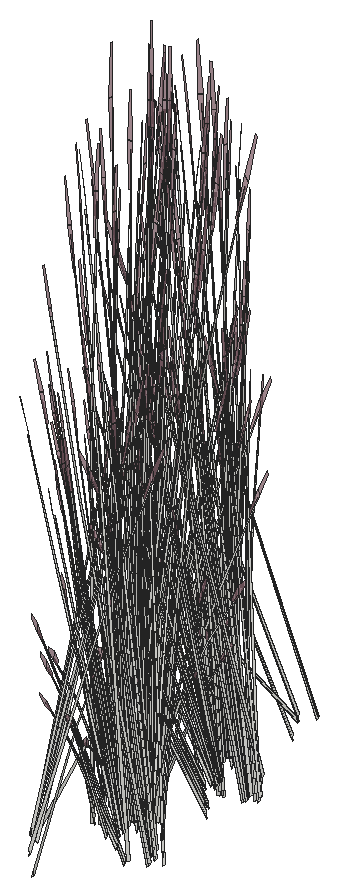
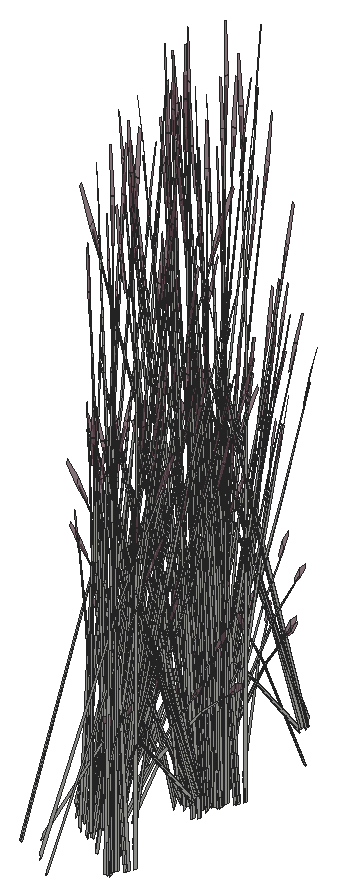
# SketchUp Ruby script. Lengths in inches.
U = 1.inch
M = Sketchup.active_model
def pt(a) = Geom::Point3d.new(a.map { |v| v * U })
def face(e, loops, mat)
  f = e.add_face(loops[0].map { |a| pt(a) })
  loops[1..].each { |l| e.add_face(l.map { |a| pt(a) }).erase! }
  f.material = f.back_material = mat if mat
  f
end
# faces: each face lists its corners as indices into pts; further lists are holes
def faces(e, pts, list, mat = nil) = list.each { |f| face(e, (f[0].is_a?(Array) ? f : [f]).map { |l| l.map { |i| pts[i] } }, mat) }
# xy, xz, yz: faces in a plane at the given z, y or x. An outline is a flat list of corners, or four numbers for a rectangle; further outlines are holes
def ring(l) = l.size == 4 ? [[l[0], l[1]], [l[2], l[1]], [l[2], l[3]], [l[0], l[3]]] : l.each_slice(2).to_a
def flat(e, list, mat, &to3) = list.each { |f| face(e, (f[0].is_a?(Array) ? f : [f]).map { |l| ring(l).map { |u, v| to3.(u, v) } }, mat) }
def xy(e, z, list, mat = nil) = flat(e, list, mat) { |x, y| [x, y, z] }
def xz(e, y, list, mat = nil) = flat(e, list, mat) { |x, z| [x, y, z] }
def yz(e, x, list, mat = nil) = flat(e, list, mat) { |y, z| [x, y, z] }
def lines(e, pts, list) = list.each { |a, b| e.add_line(pt(pts[a]), pt(pts[b])) }
# prism: a flat outline (further loops are holes) pulled along v
def prism(e, loops, v, mat = nil)
  f = face(e, loops, mat); d = Geom::Vector3d.new(v.map { |x| x * U })
  f.pushpull(f.normal.samedirection?(d) ? d.length : -d.length)
end
def box(e, o, s, mat = nil) = prism(e, [[o, [o[0] + s[0], o[1], o[2]], [o[0] + s[0], o[1] + s[1], o[2]], [o[0], o[1] + s[1], o[2]]]], [0, 0, s[2]], mat)
def at(x, y, z, deg = 0) = Geom::Transformation.translation(pt([x, y, z])) * Geom::Transformation.rotation(ORIGIN, Z_AXIS, deg.degrees)
def axes(o, x, y, z) = Geom::Transformation.new([*x, 0, *y, 0, *z, 0, *pt(o).to_a, 1])
def part(name) = M.definitions.add(name)
# library, detail: a bought-in or finely detailed component or shape, given as its bounding box
def library(name, o, s) = part(name).tap { |d| box(d.entities, o, s) }
def detail(e, o, s) = box(e.add_group.entities, o, s)
def put(e, d, t, mat = nil) = e.add_instance(d, t).tap { |i| i.material = mat if mat }
def group(e, t, mat = nil) = e.add_group.tap { |g| g.transformation = t; g.material = mat if mat }.entities
root = M.entities
M.materials.add("LightPink_Translucent").color = [144, 107, 117]
M.materials["LightPink_Translucent"].alpha = 0.75
c1 = part("blade")
p = [[2.15,0.21,22],[0,0.17,0],[0.09,0.45,0],[2.18,0.31,22],[2.29,0.31,22],[0.38,0.45,0],
  [2.48,0.24,33],[2.49,0.24,33],[2.48,0.22,33]]
faces(c1.entities,p,[[0,1,2,3],[4,5,2,3],[6,3,4,7],[8,0,3,6]])
c2 = part("seeds")
p = [[0.3,-0.1,1.38],[-0.01,-0.03,1.59],[-0.01,-0.03,0.03],[0.14,-0.07,-0.07],[0.29,-0.03,3],[0.15,0.01,3.11]]
faces(c2.entities,p,[[0,1,2,3],[1,0,4,5]],"LightPink_Translucent")
c3 = part("blade with seeds")
put(c3.entities,c1,at(0,0,0))
put(c3.entities,c2,axes([2.4,0.25,30.99],[1.5799,-0.05474,1.17369],[-0.12525,1.92788,0.29478],[-0.07173,-0.02425,1.56792]))
put(root,c3,axes([404.54,32.26,-9.59],[-0.14537,0.11002,1.33163],[-0.43536,-0.19256,-0.28638],[0.0807,-0.23948,0.56934]))
put(root,c3,axes([403.38,24.93,-7.3125],[0.50045,-0.25306,-0.11324],[0.24593,0.44915,-0.62851],[0.06603,0.18927,0.95501]))
put(root,c3,axes([408.26,29.88,-9.83],[-0.47569,0.45698,0.2864],[-0.47598,-0.45217,-0.33981],[-0.01661,-0.12977,1.53541]))
put(root,c3,axes([407.6,27.93,-7.62],[0.03791,0.05424,1.65179],[-0.18278,0.48761,-0.15608],[-0.18511,0.00353,0.29231]))
put(root,c3,axes([403.47,25.03,-10.61],[0.08277,-0.02958,1.6421],[0.49786,0.16279,-0.25086],[0.01456,0.18348,0.2797]))
put(root,c3,axes([408.12,28.9375,-7.64],[-0.37135,0.36005,-0.47583],[-0.32522,-0.38035,-0.36857],[-0.18868,-0.05478,0.91046]))
put(root,c3,axes([408.39,28.78,-7.3],[0.29098,0.34031,0.32977],[-0.33226,0.32215,-0.42575],[-0.16881,-0.04902,0.81462]))
put(root,c3,axes([407.28,29.41,-9.42],[0.3265,-0.03889,1.06958],[-0.20711,0.3427,0.78586],[-0.16135,-0.05141,0.23558]))
put(root,c3,axes([404.89,33.07,-7.36],[0.01331,-0.50278,-0.66157],[0.56035,0.03377,0.07984],[0.05914,-0.213,0.93586]))
put(root,c3,axes([403.8125,24.91,-7.64],[0.50273,0.13626,-0.47583],[-0.17232,0.46717,-0.36857],[0.0461,0.18809,0.91046]))
put(root,c3,axes([404.1,23.94,-8.39],[-0.1169,-0.17452,1.59586],[0.54019,-0.14692,0.12904],[0.12209,0.27397,0.68222]))
put(root,c3,axes([405.67,32.29,-7.61],[-0.00494,-0.10818,1.62908],[-0.41695,-0.31265,-0.25764],[0.06446,-0.18952,0.13065]))
put(root,c3,axes([405.5625,31.9,-7.62],[-0.05194,0.04152,1.65179],[-0.50886,-0.14007,-0.15608],[-0.01842,-0.18118,0.29231]))
put(root,c3,axes([408.31,28.56,-7.3125],[-0.02738,0.55277,-0.11324],[-0.51847,-0.01511,-0.62851],[-0.19968,-0.0384,0.95501]))
put(root,c3,axes([403.58,25.19,-7.78],[-0.15418,0.41799,-0.32977],[-0.44981,-0.12192,0.42575],[0.04124,0.16829,0.81462]))
put(root,c3,axes([404,31.38,-9.42],[0.06561,0.31695,1.06958],[-0.36394,-0.17555,0.78586],[0.03916,-0.16229,0.23558]))
put(root,c3,axes([404.78,32.91,-7.64],[-0.3661,-0.36521,-0.47583],[0.38674,-0.31985,-0.36857],[0.0557,-0.18556,0.91046]))
put(root,c3,axes([409.23,30.75,-10.08],[-0.53199,-0.08911,-0.58063],[0.11226,-0.54969,-0.15239],[-0.15876,-0.06661,1.28164]))
put(root,c3,axes([403.98,32.36,-7.59],[0.50393,0.1421,0.447],[-0.17232,0.46717,0.36857],[-0.03028,-0.18372,0.92496]))
put(root,c3,axes([403.63,24.82,-7.36],[0.24409,0.44196,-0.66157],[-0.50245,0.2463,0.07984],[0.05708,0.21354,0.93586]))
put(root,c3,axes([405.16,33.1,-7.3125],[-0.56206,-0.02693,-0.11324],[0.01536,-0.50991,-0.62851],[0.03904,-0.19638,0.95501]))
put(root,c3,axes([405.125,32.77,-7.78],[0.34603,-0.28618,-0.32977],[0.32756,0.32677,0.42575],[0.04984,-0.16603,0.81462]))
put(root,c3,axes([404.11,32.33,-7.6],[0.37684,-0.18473,0.05988],[0.18445,0.33686,0.47138],[-0.03639,-0.14849,0.71878]))
put(root,c3,axes([403.26,25.93,-7.61],[0.06483,0.08753,1.62908],[0.52315,0.03439,-0.25764],[0.05261,0.19303,0.13065]))
put(root,c3,axes([407.57,29.72,-7.59],[0.14449,-0.4956,0.447],[0.47502,0.16947,0.36857],[-0.1868,0.02978,0.92496]))
put(root,c3,axes([407.53,29.59,-7.6],[-0.18783,-0.37061,0.05988],[0.34252,-0.1814,0.47138],[-0.15099,0.03579,0.71878]))
put(root,c3,axes([407.52,29.97,-10.61],[0.01297,0.08566,1.6421],[-0.26146,0.44735,-0.25086],[-0.18572,-0.02255,0.2797]))
put(root,c3,axes([408.67,31.59,-10.11],[-0.12013,-0.47362,-0.28847],[0.47712,-0.13449,0.28847],[-0.09619,-0.05462,1.29413]))
put(root,c3,axes([408.53,31.79,-10.12],[-0.47863,-0.27177,-0.46235],[0.28609,-0.48733,0],[-0.10901,-0.0619,1.46668]))
put(root,c3,axes([409.83,30.83,-9.52],[-0.51635,0.36087,-0.27094],[-0.34336,-0.5099,-0.46562],[-0.1274,-0.05178,1.4872]))
put(root,c3,axes([405.125,32.88,-7.59],[0.36417,0.37086,0.447],[-0.38674,0.31985,0.36857],[0.06718,-0.174,0.92496]))
put(root,c3,axes([405.26,32.92,-7.6],[0.42027,0.02533,0.05988],[-0.01152,0.38243,0.47138],[0.04398,-0.14649,0.71878]))
put(root,c3,axes([404.94,33.18,-7.3],[-0.34603,0.28618,0.32977],[-0.32756,-0.32677,-0.42575],[0.04984,-0.16603,0.81462]))
put(root,c3,axes([402.67,32.7,-9.79],[-0.31974,-0.54466,0],[0.53494,-0.30375,-0.48057],[0.12184,-0.06918,1.52448]))
put(root,c3,axes([407.92,29.73,-7.3],[0.42502,0.15163,0.32977],[-0.12396,0.44238,-0.42575],[-0.17112,0.04056,0.81462]))
put(root,c3,axes([403.1,32.62,-10.12],[0.47863,-0.27177,-0.46235],[0.28609,0.48733,0],[0.10901,-0.0619,1.46668]))
put(root,c3,axes([403.67,33.73,-10.08],[0.34446,-0.40855,-0.58063],[0.42791,0.37046,-0.15239],[0.13803,-0.10191,1.28164]))
put(root,c3,axes([407.76,30,-7.64],[-0.13855,0.49442,-0.47583],[-0.47502,-0.16947,-0.36857],[-0.19125,0.04534,0.91046]))
put(root,c3,axes([407.74,29.58,-7.3125],[0.25732,0.49218,-0.11324],[-0.45669,0.24187,-0.62851],[-0.19245,0.06494,0.95501]))
put(root,c3,axes([408.82,32.12,-9.79],[-0.31974,0.54466,0],[-0.53494,-0.30375,-0.48057],[-0.12184,-0.06918,1.52448]))
put(root,c3,axes([403.29,34.2,-9.52],[-0.05959,-0.62022,-0.27094],[0.62068,-0.0375,-0.46562],[0.1093,-0.08261,1.4872]))
put(root,c3,axes([405.54,34.0625,-7.3],[-0.44516,0.07768,0.32977],[-0.11755,-0.44407,-0.42575],[0.12757,-0.11927,0.81462]))
put(root,c3,axes([403.21,32.83,-10.11],[0.47712,0.13449,-0.28847],[-0.12013,0.47362,0.28847],[0.09619,-0.05462,1.29413]))
put(root,c3,axes([407.68,30.96,-7.59],[-0.12683,-0.50025,0.447],[0.49754,-0.08682,0.36857],[-0.14663,0.11765,0.92496]))
put(root,c3,axes([407.58,30.86,-7.6],[-0.35109,-0.22859,0.05988],[0.2044,-0.32553,0.47138],[-0.11256,0.10524,0.71878]))
put(root,c3,axes([403.375,34.69,-9.73],[0.57623,0.26344,0.22409],[-0.27732,0.5474,0.46562],[0,-0.12618,1.49497]))
put(root,c3,axes([407.99,30.79,-7.3],[0.44516,-0.07768,0.32977],[0.11755,0.44407,-0.42575],[-0.12757,0.11927,0.81462]))
put(root,c3,axes([406.27,30.59,-7.62],[0.06527,0.01458,1.65179],[0.20191,0.48025,-0.15608],[-0.1336,0.12605,0.29231]))
put(root,c3,axes([406.82,32.12,-9.42],[0.21313,-0.24635,1.06958],[0.0841,0.38999,0.78586],[-0.15402,0.06983,0.23558]))
put(root,c3,axes([407.625,31.05,-7.78],[-0.44516,0.07768,-0.32977],[-0.11755,-0.44407,0.42575],[-0.12757,0.11927,0.81462]))
put(root,c3,axes([403.1875,34.32,-9.47],[-0.55535,0.03355,0.41661],[-0.05022,-0.55698,-0.2005],[0.09942,-0.05645,1.33761]))
put(root,c3,axes([406.98,32.05,-6.74],[0.45129,0.14509,-0.06041],[-0.13882,0.44656,-0.27392],[-0.07381,0.0678,0.90349]))
put(root,c3,axes([410.18,31.22,-10.08],[-0.34446,0.40855,-0.58063],[-0.42791,-0.37046,-0.15239],[-0.13803,0.10191,1.28164]))
put(root,c3,axes([403.97,34.57,-9.95],[0,-0.62892,0],[0.63949,0,0],[0,0,1.6711]))
put(root,c3,axes([404.75,33.12,-9.69],[-0.47863,-0.27177,0.46235],[0.28609,-0.48733,0],[0.10901,0.0619,1.46668]))
put(root,c3,axes([403.67,34.18,-9.8],[-0.42403,0.49328,0.42607],[-0.50377,-0.43543,0.16719],[0.10223,-0.04923,1.47927]))
put(root,c3,axes([407.76,30.75,-7.3125],[0.47307,0.29971,-0.11324],[-0.27254,0.43404,-0.62851],[-0.13365,0.15087,0.95501]))
put(root,c3,axes([402.93,33.37,-9.7],[-0.14774,0.54019,0.16428],[-0.54062,-0.15287,0.32672],[0.09339,-0.00263,1.49371]))
put(root,c3,axes([408.36,38.75,-8.39],[0.1169,0.17452,1.59586],[-0.54019,0.14692,0.12904],[-0.12209,-0.27397,0.68222]))
put(root,c3,axes([408.39,30.62,-8.39],[0.12773,-0.16701,1.59586],[0.32252,0.4508,0.12904],[-0.22121,0.20529,0.68222]))
put(root,c3,axes([404.06,33.97,-9.5625],[0.09866,-0.48509,0.13483],[0.48202,0.0842,-0.38503],[0.08772,0.04981,1.18024]))
put(root,c3,axes([407.99,31.11,-7.64],[0.13138,0.49631,-0.47583],[-0.49754,0.08682,-0.36857],[-0.14258,0.13331,0.91046]))
put(root,c3,axes([403.85,34.09,-9.47],[-0.30722,-0.45622,0.41661],[0.46535,-0.32126,-0.2005],[0.09942,0.05645,1.33761]))
put(root,c3,axes([408.21,38.28,-9.59],[-0.03097,0.17781,1.33163],[-0.45273,0.14885,-0.28638],[-0.10583,-0.22982,0.56934]))
put(root,c3,axes([408.27,31.94,-7.6],[-0.42027,-0.02533,0.05988],[0.01152,-0.38243,0.47138],[-0.04398,0.14649,0.71878]))
put(root,c3,axes([407.38,32.37,-10.61],[0.0686,0.0543,1.6421],[0.11632,0.50315,-0.25086],[-0.15204,0.10729,0.2797]))
put(root,c3,axes([408.41,31.97,-7.59],[-0.36417,-0.37086,0.447],[0.38674,-0.31985,0.36857],[-0.06718,0.174,0.92496]))
put(root,c3,axes([404.01,34.125,-9.52],[0.51635,-0.36087,-0.27094],[0.34336,0.5099,-0.46562],[0.1274,0.05178,1.4872]))
put(root,c3,axes([404.4,34.72,-9.95],[0.57217,0,0],[0,0.56272,0],[0,0,1.66132]))
put(root,c3,axes([404.57,33.4,-9.7],[-0.54955,0.14427,0.16428],[-0.1357,-0.53689,0.32672],[0.04901,0.07823,1.49371]))
put(root,c3,axes([405.18,33.37,-10.11],[0.12013,0.47362,-0.28847],[-0.47712,0.13449,0.28847],[0.09619,0.05462,1.29413]))
put(root,c3,axes([408.3,31.03,-8.39],[0.09522,-0.18683,1.59586],[0.39947,0.38663,0.12904],[-0.18021,0.24097,0.68222]))
put(root,c3,axes([404.22,34.43,-9.78],[-0.64638,-0.11452,0.45814],[0.13155,-0.64678,0.17978],[0.09446,0.06245,1.59061]))
put(root,c3,axes([408.72,37.34,-7.62],[-0.00954,0.06515,1.65179],[-0.47055,0.23645,-0.15608],[-0.13847,-0.12087,0.29231]))
put(root,c3,axes([408.41,32.08,-7.78],[-0.34603,0.28618,-0.32977],[-0.32756,-0.32677,0.42575],[-0.04984,0.16603,0.81462]))
put(root,c3,axes([407.21,32,-7.61],[-0.01271,0.10756,1.62908],[0.36076,0.37419,-0.25764],[-0.09444,0.17695,0.13065]))
put(root,c3,axes([404.33,35.96,-9.97],[0.53691,-0.18442,-0.17877],[0.18866,0.53125,0.00007],[0.05927,-0.02038,1.61933]))
put(root,c3,axes([408.62,38.49,-7.26],[0.56969,-0.13971,0.50064],[0.09887,0.54803,0.4128],[-0.13398,-0.16152,1.03595]))
put(root,c3,axes([404.39,34.96,-9.9375],[0.35699,0.35109,0],[-0.35699,0.35109,0],[0,0,1.57621]))
put(root,c3,axes([405.36,34.8,-9.7],[-0.40181,-0.39593,0.16428],[0.40492,-0.38402,0.32672],[-0.04438,0.08086,1.49371]))
put(root,c3,axes([408.06,38,-9.42],[0.26677,0.18918,1.06958],[-0.38851,0.11372,0.78586],[-0.08313,-0.14539,0.23558]))
put(root,c3,axes([408.7,39,-7.36],[-0.43608,-0.26272,-0.66157],[0.30991,-0.46038,0.07984],[-0.158,-0.15687,0.93586]))
put(root,c3,axes([408.55,38.65,-7.78],[-0.07899,-0.43781,-0.32977],[0.45153,-0.11561,0.42575],[-0.12128,-0.12546,0.81462]))
put(root,c3,axes([404.39,34.55,-9.47],[0.24813,-0.48978,0.41661],[0.51557,0.23571,-0.2005],[0,0.1129,1.33761]))
put(root,c3,axes([404.29,34.83,-9.87],[0,0.62861,-0.05249],[-0.63949,0,0],[0,0.01975,1.67027]))
put(root,c3,axes([404.34,34.38,-9.94],[0.30722,0.45622,-0.41661],[-0.46535,0.32126,0.2005],[0.09942,0.05645,1.33761]))
put(root,c3,axes([408.75,38.61,-7.6],[0.23243,-0.34529,0.05988],[0.331,0.20103,0.47138],[-0.10701,-0.1107,0.71878]))
put(root,c3,axes([407.85,38.57,-10.61],[-0.04954,0.0716,1.6421],[-0.50062,0.15438,-0.25086],[-0.12094,-0.14044,0.2797]))
put(root,c3,axes([405.6875,34.82,-9.69],[0,-0.54355,0.46235],[0.57217,0,0],[0,0.1238,1.46668]))
put(root,c3,axes([404.6,34.66,-9.5625],[0.47648,-0.15851,0.13483],[0.16686,0.45265,-0.38503],[0,0.09962,1.18024]))
put(root,c3,axes([407.17,33.1,-7.62],[0.05802,-0.03282,1.65179],[0.47954,0.21828,-0.15608],[-0.01127,0.18175,0.29231]))
put(root,c3,axes([408.5,39.01,-7.64],[-0.50465,0.12921,-0.47583],[-0.08828,-0.48932,-0.36857],[-0.13555,-0.14022,0.91046]))
put(root,c3,axes([408.85,38.58,-6.94],[-0.34131,0.52108,-0.12682],[-0.49429,-0.3002,-0.70393],[-0.17182,-0.14722,1.06961]))
put(root,c3,axes([404.17,36.25,-9.95],[0.51557,0.24403,0],[-0.24813,0.50705,0],[0,0,1.62917]))
put(root,c3,axes([408.24,32.91,-9.59],[0.16138,-0.08575,1.33163],[0.39845,0.25854,-0.28638],[-0.1186,0.22371,0.56934]))
put(root,c3,axes([407.54,38.43,-7.61],[-0.11004,-0.00384,1.62908],[-0.35032,0.38367,-0.25764],[-0.18692,-0.07839,0.13065]))
put(root,c3,axes([409.75,41.97,-8.9],[0.44194,0.21918,1.40854],[-0.43295,0.47219,0.557],[-0.19393,-0.27986,1.18082]))
put(root,c3,axes([403.99,36.04,-9.87],[0.22235,0.62444,-0.05599],[-0.63531,0.21881,0],[0.00776,0.02181,1.60327]))
put(root,c3,axes([408.82,39.01,-7.3],[0.07899,0.43781,0.32977],[-0.45153,0.11561,-0.42575],[-0.12128,-0.12546,0.81462]))
put(root,c3,axes([407.46,39.3,-7.26],[0.42234,-0.40113,0.50064],[0.36424,0.42599,0.4128],[-0.19815,-0.07399,1.03595]))
put(root,c3,axes([406.08,34.91,-9.79],[0.63949,0,0],[0,0.60749,-0.48057],[0,0.13836,1.52448]))
put(root,c3,axes([405.82,35.22,-9.95],[-0.63917,-0.00435,-0.04634],[0,-0.60749,0.46507],[-0.02009,0.13829,1.47457]))
put(root,c3,axes([404.4375,34.69,-9.52],[0.57594,0.25935,-0.27094],[-0.27732,0.5474,-0.46562],[0.0181,0.1344,1.4872]))
put(root,c3,axes([405.6875,35.3125,-10.11],[-0.35699,0.33913,-0.28847],[-0.35699,-0.33913,0.28847],[0,0.10923,1.29413]))
put(root,c3,axes([404.375,35.1,-9.94],[-0.24813,0.48978,-0.41661],[-0.51557,-0.23571,0.2005],[0,0.1129,1.33761]))
put(root,c3,axes([407.65,39.29,-7.6],[0.02575,-0.41332,0.05988],[0.38885,0.01133,0.47138],[-0.14895,-0.04325,0.71878]))
put(root,c3,axes([407.51,39.42,-7.78],[-0.29098,-0.34031,-0.32977],[0.33226,-0.32215,0.42575],[-0.16881,-0.04902,0.81462]))
put(root,c3,axes([407.54,38.84,-10.02],[-0.14753,0.44383,-0.03625],[-0.45406,-0.13653,-0.16435],[-0.06894,-0.07259,0.54209]))
put(root,c3,axes([407.29,40.87,-9.79],[-0.63949,0,0],[0,-0.60749,-0.48057],[0,-0.13836,1.52448]))
put(root,c3,axes([404.24,36.67,-7.3],[-0.07899,-0.43781,0.32977],[0.45153,-0.11561,-0.42575],[0.12128,0.12546,0.81462]))
put(root,c3,axes([405.93,35.32,-10.12],[0,0.54355,-0.46235],[-0.57217,0,0],[0,0.1238,1.46668]))
put(root,c3,axes([404.54,34.15,-7.83],[-0.44191,-0.28242,1.28769],[0.46662,-0.43971,0.5556],[0.14258,0.26499,1.24467]))
put(root,c3,axes([405.21,36.45,-9.42],[-0.28795,-0.15629,1.06958],[0.37181,-0.1588,0.78586],[0.10029,0.13452,0.23558]))
put(root,c3,axes([407.79,40.71,-9.83],[-0.47569,0.45698,0.2864],[-0.47598,-0.45217,-0.33981],[-0.01661,-0.12977,1.53541]))
put(root,c3,axes([403.8,37.28,-7.62],[0.00151,-0.06581,1.65179],[0.43826,-0.29033,-0.15608],[0.15223,0.10363,0.29231]))
put(root,c3,axes([404.67,35.25,-10.05],[0.18752,0.49766,-0.6445],[-0.54017,0.17923,-0.16915],[0.02073,0.16852,1.42262]))
put(root,c3,axes([403.16,36.74,-7.3],[0.15418,-0.41799,0.32977],[0.44981,0.12192,-0.42575],[0.04124,0.16829,0.81462]))
put(root,c3,axes([407.92,39.6,-7.3],[0.29098,0.34031,0.32977],[-0.33226,0.32215,-0.42575],[-0.16881,-0.04902,0.81462]))
put(root,c3,axes([406.81,40.24,-9.42],[0.3265,-0.03889,1.06958],[-0.20711,0.3427,0.78586],[-0.16135,-0.05141,0.23558]))
put(root,c3,axes([405.25,37.16,-9.52],[-0.32795,-0.01705,0.97832],[0.21658,-0.36206,0.54015],[0.12956,0.12863,0.76741]))
put(root,c3,axes([407.84,39.38,-7.3125],[-0.02738,0.55277,-0.11324],[-0.51847,-0.01511,-0.62851],[-0.19968,-0.0384,0.95501]))
put(root,c3,axes([404.31,37.07,-7.6],[-0.23243,0.34529,0.05988],[-0.331,-0.20103,0.47138],[0.10701,0.1107,0.71878]))
put(root,c3,axes([403.76,38.23,-6.74],[0.35341,-0.31182,-0.06041],[0.32382,0.34152,-0.27392],[0.0228,0.09677,0.90349]))
put(root,c3,axes([409.03,41.4,-9.94],[-0.30722,-0.45622,-0.41661],[0.46535,-0.32126,0.2005],[-0.09942,-0.05645,1.33761]))
put(root,c3,axes([404.41,36.97,-7.59],[-0.50866,0.12474,0.447],[-0.08828,-0.48932,0.36857],[0.11963,0.14421,0.92496]))
put(root,c3,axes([404.18,36.28,-9.59],[0.00902,-0.18018,1.33163],[0.43127,-0.20126,-0.28638],[0.13313,0.21566,0.56934]))
put(root,c3,axes([404.5625,44.12,-9.59],[-0.14537,0.11002,1.33163],[-0.43536,-0.19256,-0.28638],[0.0807,-0.23948,0.56934]))
put(root,c3,axes([403.01,36.92,-7.3125],[0.50045,-0.25306,-0.11324],[0.24593,0.44915,-0.62851],[0.06603,0.18927,0.95501]))
put(root,c3,axes([408.76,41.58,-10.08],[-0.53199,-0.08911,-0.58063],[0.11226,-0.54969,-0.15239],[-0.15876,-0.06661,1.28164]))
put(root,c3,axes([404.92,44.93,-7.36],[0.01331,-0.50278,-0.66157],[0.56035,0.03377,0.07984],[0.05914,-0.213,0.93586]))
put(root,c3,axes([407.09,40.55,-7.59],[0.14449,-0.4956,0.447],[0.47502,0.16947,0.36857],[-0.1868,0.02978,0.92496]))
put(root,c3,axes([407.05,40.42,-7.6],[-0.18783,-0.37061,0.05988],[0.34252,-0.1814,0.47138],[-0.15099,0.03579,0.71878]))
put(root,c3,axes([405.7,44.15,-7.61],[-0.00494,-0.10818,1.62908],[-0.41695,-0.31265,-0.25764],[0.06446,-0.18952,0.13065]))
put(root,c3,axes([405.59,43.76,-7.62],[-0.05194,0.04152,1.65179],[-0.50886,-0.14007,-0.15608],[-0.01842,-0.18118,0.29231]))
put(root,c3,axes([403.4375,36.89,-7.64],[0.50273,0.13626,-0.47583],[-0.17232,0.46717,-0.36857],[0.0461,0.18809,0.91046]))
put(root,c3,axes([403.72,35.93,-8.39],[-0.1169,-0.17452,1.59586],[0.54019,-0.14692,0.12904],[0.12209,0.27397,0.68222]))
put(root,c3,axes([408.19,42.41,-10.11],[-0.12013,-0.47362,-0.28847],[0.47712,-0.13449,0.28847],[-0.09619,-0.05462,1.29413]))
put(root,c3,axes([404.03,43.24,-9.42],[0.06561,0.31695,1.06958],[-0.36394,-0.17555,0.78586],[0.03916,-0.16229,0.23558]))
put(root,c3,axes([404.8,44.77,-7.64],[-0.3661,-0.36521,-0.47583],[0.38674,-0.31985,-0.36857],[0.0557,-0.18556,0.91046]))
put(root,c3,axes([408.06,42.62,-10.12],[-0.47863,-0.27177,-0.46235],[0.28609,-0.48733,0],[-0.10901,-0.0619,1.46668]))
put(root,c3,axes([409.36,41.66,-9.52],[-0.51635,0.36087,-0.27094],[-0.34336,-0.5099,-0.46562],[-0.1274,-0.05178,1.4872]))
put(root,c3,axes([404,44.22,-7.59],[0.50393,0.1421,0.447],[-0.17232,0.46717,0.36857],[-0.03028,-0.18372,0.92496]))
put(root,c3,axes([405.1875,44.96,-7.3125],[-0.56206,-0.02693,-0.11324],[0.01536,-0.50991,-0.62851],[0.03904,-0.19638,0.95501]))
put(root,c3,axes([405.15,44.63,-7.78],[0.34603,-0.28618,-0.32977],[0.32756,0.32677,0.42575],[0.04984,-0.16603,0.81462]))
put(root,c3,axes([404.14,44.1875,-7.6],[0.37684,-0.18473,0.05988],[0.18445,0.33686,0.47138],[-0.03639,-0.14849,0.71878]))
put(root,c3,axes([403.25,36.8,-7.36],[0.24409,0.44196,-0.66157],[-0.50245,0.2463,0.07984],[0.05708,0.21354,0.93586]))
put(root,c3,axes([402.89,37.92,-7.61],[0.06483,0.08753,1.62908],[0.52315,0.03439,-0.25764],[0.05261,0.19303,0.13065]))
put(root,c3,axes([407.44,40.56,-7.3],[0.42502,0.15163,0.32977],[-0.12396,0.44238,-0.42575],[-0.17112,0.04056,0.81462]))
put(root,c3,axes([409.9375,41.82,-9.7],[-0.49938,-0.43748,-0.23459],[0.42021,-0.49126,0.51337],[-0.13447,0.05118,1.56642]))
put(root,c3,axes([405.15,44.74,-7.59],[0.36417,0.37086,0.447],[-0.38674,0.31985,0.36857],[0.06718,-0.174,0.92496]))
put(root,c3,axes([405.28,44.78,-7.6],[0.42027,0.02533,0.05988],[-0.01152,0.38243,0.47138],[0.04398,-0.14649,0.71878]))
put(root,c3,axes([407.26,40.41,-7.3125],[0.25732,0.49218,-0.11324],[-0.45669,0.24187,-0.62851],[-0.19245,0.06494,0.95501]))
put(root,c3,axes([404.97,45.04,-7.3],[-0.34603,0.28618,0.32977],[-0.32756,-0.32677,-0.42575],[0.04984,-0.16603,0.81462]))
put(root,c3,axes([408.35,42.94,-9.79],[-0.31974,0.54466,0],[-0.53494,-0.30375,-0.48057],[-0.12184,-0.06918,1.52448]))
put(root,c3,axes([402.6875,44.56,-9.79],[-0.31974,-0.54466,0],[0.53494,-0.30375,-0.48057],[0.12184,-0.06918,1.52448]))
put(root,c3,axes([409.6875,41.73,-9.94],[-0.55535,0.03355,-0.41661],[-0.05022,-0.55698,0.2005],[-0.09942,0.05645,1.33761]))
put(root,c3,axes([403.12,44.47,-10.12],[0.47863,-0.27177,-0.46235],[0.28609,0.48733,0],[0.10901,-0.0619,1.46668]))
put(root,c3,axes([407.21,41.78,-7.59],[-0.12683,-0.50025,0.447],[0.49754,-0.08682,0.36857],[-0.14663,0.11765,0.92496]))
put(root,c3,axes([407.11,41.6875,-7.6],[-0.35109,-0.22859,0.05988],[0.2044,-0.32553,0.47138],[-0.11256,0.10524,0.71878]))
put(root,c3,axes([403.69,45.59,-10.08],[0.34446,-0.40855,-0.58063],[0.42791,0.37046,-0.15239],[0.13803,-0.10191,1.28164]))
put(root,c3,axes([403.32,46.0625,-9.52],[-0.05959,-0.62022,-0.27094],[0.62068,-0.0375,-0.46562],[0.1093,-0.08261,1.4872]))
put(root,c3,axes([407.51,41.62,-7.3],[0.44516,-0.07768,0.32977],[0.11755,0.44407,-0.42575],[-0.12757,0.11927,0.81462]))
put(root,c3,axes([405.57,45.92,-7.3],[-0.44516,0.07768,0.32977],[-0.11755,-0.44407,-0.42575],[0.12757,-0.11927,0.81462]))
put(root,c3,axes([406.34,42.95,-9.42],[0.21313,-0.24635,1.06958],[0.0841,0.38999,0.78586],[-0.15402,0.06983,0.23558]))
put(root,c3,axes([403.23,44.6875,-10.11],[0.47712,0.13449,-0.28847],[-0.12013,0.47362,0.28847],[0.09619,-0.05462,1.29413]))
put(root,c3,axes([407.15,41.88,-7.78],[-0.44516,0.07768,-0.32977],[-0.11755,-0.44407,0.42575],[-0.12757,0.11927,0.81462]))
put(root,c3,axes([406.5,42.88,-6.74],[0.45129,0.14509,-0.06041],[-0.13882,0.44656,-0.27392],[-0.07381,0.0678,0.90349]))
put(root,c3,axes([409.7,42.05,-10.08],[-0.34446,0.40855,-0.58063],[-0.42791,-0.37046,-0.15239],[-0.13803,0.10191,1.28164]))
put(root,c3,axes([403.4,46.55,-9.73],[0.57623,0.26344,0.22409],[-0.27732,0.5474,0.46562],[0,-0.12618,1.49497]))
put(root,c3,axes([407.28,41.58,-7.3125],[0.47307,0.29971,-0.11324],[-0.27254,0.43404,-0.62851],[-0.13365,0.15087,0.95501]))
put(root,c3,axes([406.95,49.57,-8.39],[0.1169,0.17452,1.59586],[-0.54019,0.14692,0.12904],[-0.12209,-0.27397,0.68222]))
put(root,c3,axes([407.92,41.44,-8.39],[0.12773,-0.16701,1.59586],[0.32252,0.4508,0.12904],[-0.22121,0.20529,0.68222]))
put(root,c3,axes([407.84,48.42,-7.61],[-0.07822,-0.07621,1.62908],[-0.52201,0.04832,-0.25764],[-0.08331,-0.18228,0.13065]))
put(root,c3,axes([407.51,41.93,-7.64],[0.13138,0.49631,-0.47583],[-0.49754,0.08682,-0.36857],[-0.14258,0.13331,0.91046]))
put(root,c3,axes([403.21,46.18,-9.47],[-0.55535,0.03355,0.41661],[-0.05022,-0.55698,-0.2005],[0.09942,-0.05645,1.33761]))
put(root,c3,axes([408.39,49.71,-7.36],[-0.24409,-0.44196,-0.66157],[0.50245,-0.2463,0.07984],[-0.05708,-0.21354,0.93586]))
put(root,c3,axes([406.8,49.11,-9.59],[-0.03097,0.17781,1.33163],[-0.45273,0.14885,-0.28638],[-0.10583,-0.22982,0.56934]))
put(root,c3,axes([407.8,42.76,-7.6],[-0.42027,-0.02533,0.05988],[0.01152,-0.38243,0.47138],[-0.04398,0.14649,0.71878]))
put(root,c3,axes([406.9,43.2,-10.61],[0.0686,0.0543,1.6421],[0.11632,0.50315,-0.25086],[-0.15204,0.10729,0.2797]))
